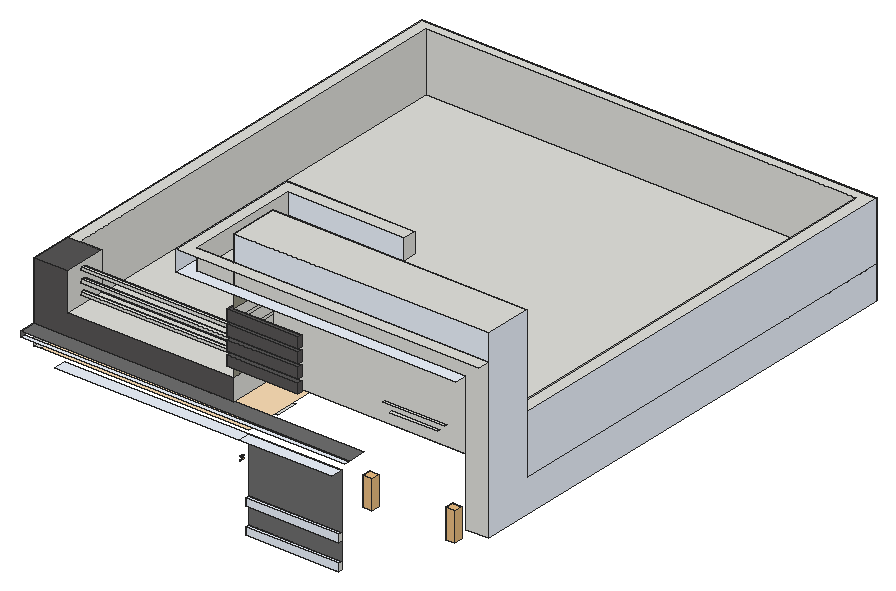
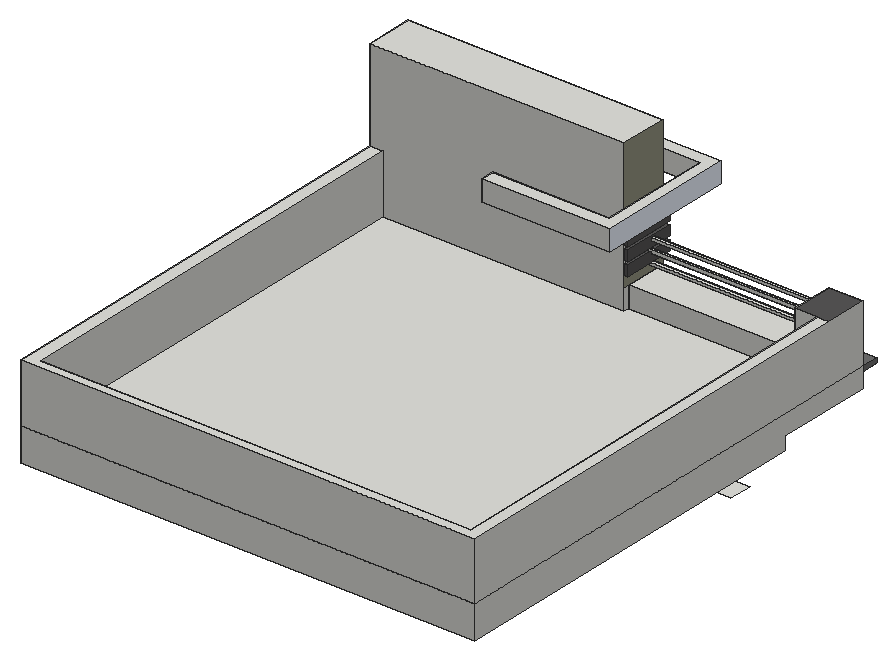
# SketchUp Ruby script. Lengths in inches.
U = 1.inch
M = Sketchup.active_model
def pt(a) = Geom::Point3d.new(a.map { |v| v * U })
def face(e, loops, mat)
  f = e.add_face(loops[0].map { |a| pt(a) })
  loops[1..].each { |l| e.add_face(l.map { |a| pt(a) }).erase! }
  f.material = f.back_material = mat if mat
  f
end
# faces: each face lists its corners as indices into pts; further lists are holes
def faces(e, pts, list, mat = nil) = list.each { |f| face(e, (f[0].is_a?(Array) ? f : [f]).map { |l| l.map { |i| pts[i] } }, mat) }
# xy, xz, yz: faces in a plane at the given z, y or x. An outline is a flat list of corners, or four numbers for a rectangle; further outlines are holes
def ring(l) = l.size == 4 ? [[l[0], l[1]], [l[2], l[1]], [l[2], l[3]], [l[0], l[3]]] : l.each_slice(2).to_a
def flat(e, list, mat, &to3) = list.each { |f| face(e, (f[0].is_a?(Array) ? f : [f]).map { |l| ring(l).map { |u, v| to3.(u, v) } }, mat) }
def xy(e, z, list, mat = nil) = flat(e, list, mat) { |x, y| [x, y, z] }
def xz(e, y, list, mat = nil) = flat(e, list, mat) { |x, z| [x, y, z] }
def yz(e, x, list, mat = nil) = flat(e, list, mat) { |y, z| [x, y, z] }
def lines(e, pts, list) = list.each { |a, b| e.add_line(pt(pts[a]), pt(pts[b])) }
# prism: a flat outline (further loops are holes) pulled along v
def prism(e, loops, v, mat = nil)
  f = face(e, loops, mat); d = Geom::Vector3d.new(v.map { |x| x * U })
  f.pushpull(f.normal.samedirection?(d) ? d.length : -d.length)
end
def box(e, o, s, mat = nil) = prism(e, [[o, [o[0] + s[0], o[1], o[2]], [o[0] + s[0], o[1] + s[1], o[2]], [o[0], o[1] + s[1], o[2]]]], [0, 0, s[2]], mat)
def at(x, y, z, deg = 0) = Geom::Transformation.translation(pt([x, y, z])) * Geom::Transformation.rotation(ORIGIN, Z_AXIS, deg.degrees)
def axes(o, x, y, z) = Geom::Transformation.new([*x, 0, *y, 0, *z, 0, *pt(o).to_a, 1])
def part(name) = M.definitions.add(name)
# library, detail: a bought-in or finely detailed component or shape, given as its bounding box
def library(name, o, s) = part(name).tap { |d| box(d.entities, o, s) }
def detail(e, o, s) = box(e.add_group.entities, o, s)
def put(e, d, t, mat = nil) = e.add_instance(d, t).tap { |i| i.material = mat if mat }
def group(e, t, mat = nil) = e.add_group.tap { |g| g.transformation = t; g.material = mat if mat }.entities
root = M.entities
M.materials.add("Generic").color = [111, 111, 111]
M.materials.add("Generic\#1").color = [88, 86, 86]
M.materials.add("Generic\#2").color = [253, 222, 182]
M.materials.add("Generic\#3").color = [151, 150, 132]
M.materials.add("Generic\#4").color = [238, 245, 255]
M.materials.add("Generic\#5").color = [7, 6, 6]
M.materials.add("Material \#1").color = [140, 140, 140]
c1 = library("3DGeom~14_Defintion",[-102.17,352.37,-727.27],[204.35,204.35,1000])
c2 = library("3DGeom~1_Defintion",[-60.87,347.29,-704.08],[121.74,121.75,1000])
c3 = library("Lamp Wall Outdoor 94-02",[-1.89,-4.65,-3.17],[3.78,4.65,6.35])
xy(root,197.069,[[128.435,116.314,128.381,116.332,128.4375,116.329],[128.435,116.314,128.4375,116.329,128.489,116.329],[128.435,116.314,128.489,116.329,128.492,116.314],[128.492,116.314,128.489,116.329,128.537,116.346],[128.492,116.314,128.537,116.346,128.545,116.332],
  [128.4375,116.329,128.381,116.332,128.389,116.346],[128.381,116.332,128.337,116.367,128.389,116.346],[128.545,116.332,128.537,116.346,128.576,116.377],[128.545,116.332,128.576,116.377,128.589,116.367],[128.389,116.346,128.337,116.367,128.35,116.377],
  [128.337,116.367,128.309,116.413,128.35,116.377],[128.589,116.367,128.576,116.377,128.602,116.418],[128.589,116.367,128.602,116.418,128.617,116.413],[128.35,116.377,128.309,116.413,128.324,116.418],[128.309,116.413,128.299,116.465,128.324,116.418],
  [128.617,116.413,128.602,116.418,128.611,116.465],[128.617,116.413,128.611,116.465,128.627,116.465],[128.324,116.418,128.299,116.465,128.315,116.465],[128.299,116.465,128.309,116.518,128.315,116.465],[128.315,116.465,128.309,116.518,128.324,116.513],
  [128.611,116.465,128.602,116.513,128.627,116.465],[128.627,116.465,128.602,116.513,128.617,116.518],[128.324,116.513,128.309,116.518,128.337,116.564],[128.324,116.513,128.337,116.564,128.35,116.554],[128.602,116.513,128.576,116.554,128.617,116.518],
  [128.617,116.518,128.576,116.554,128.589,116.564],[128.35,116.554,128.337,116.564,128.381,116.598],[128.35,116.554,128.381,116.598,128.389,116.585],[128.576,116.554,128.537,116.585,128.589,116.564],[128.589,116.564,128.537,116.585,128.545,116.598],
  [128.389,116.585,128.381,116.598,128.435,116.616],[128.389,116.585,128.435,116.616,128.4375,116.601],[128.537,116.585,128.489,116.601,128.545,116.598],[128.545,116.598,128.489,116.601,128.492,116.616],[128.4375,116.601,128.435,116.616,128.492,116.616],
  [128.4375,116.601,128.492,116.616,128.489,116.601]],"Material \#1")
xy(root,197.085,[[128.435,116.314,128.389,116.346,128.381,116.332],[128.435,116.314,128.4375,116.329,128.389,116.346],[128.435,116.314,128.492,116.314,128.4375,116.329],[128.492,116.314,128.489,116.329,128.4375,116.329],[128.492,116.314,128.545,116.332,128.489,116.329],
  [128.489,116.329,128.545,116.332,128.537,116.346],[128.381,116.332,128.35,116.377,128.337,116.367],[128.381,116.332,128.389,116.346,128.35,116.377],[128.545,116.332,128.589,116.367,128.537,116.346],[128.537,116.346,128.589,116.367,128.576,116.377],
  [128.337,116.367,128.324,116.418,128.309,116.413],[128.337,116.367,128.35,116.377,128.324,116.418],[128.589,116.367,128.617,116.413,128.576,116.377],[128.576,116.377,128.617,116.413,128.602,116.418],[128.309,116.413,128.315,116.465,128.299,116.465],
  [128.309,116.413,128.324,116.418,128.315,116.465],[128.617,116.413,128.627,116.465,128.602,116.418],[128.602,116.418,128.627,116.465,128.611,116.465],[128.299,116.465,128.315,116.465,128.324,116.513],[128.299,116.465,128.324,116.513,128.309,116.518],
  [128.611,116.465,128.617,116.518,128.602,116.513],[128.611,116.465,128.627,116.465,128.617,116.518],[128.324,116.513,128.35,116.554,128.309,116.518],[128.602,116.513,128.589,116.564,128.576,116.554],[128.602,116.513,128.617,116.518,128.589,116.564],
  [128.309,116.518,128.35,116.554,128.337,116.564],[128.35,116.554,128.389,116.585,128.337,116.564],[128.576,116.554,128.545,116.598,128.537,116.585],[128.576,116.554,128.589,116.564,128.545,116.598],[128.337,116.564,128.389,116.585,128.381,116.598],
  [128.389,116.585,128.4375,116.601,128.381,116.598],[128.537,116.585,128.492,116.616,128.489,116.601],[128.537,116.585,128.545,116.598,128.492,116.616],[128.381,116.598,128.4375,116.601,128.435,116.616],[128.4375,116.601,128.489,116.601,128.435,116.616],
  [128.489,116.601,128.492,116.616,128.435,116.616]],"Material \#1")
xy(root,203.189,[[169.979,34.653,243.692,37.591]],"Generic\#4")
xy(root,209.126,[[169.979,34.653,243.692,37.591]],"Generic\#4")
xy(root,223.751,[[169.979,34.653,243.692,37.591]],"Generic\#4")
xy(root,228.434,[[128.435,116.314,128.381,116.332,128.389,116.346],[128.435,116.314,128.389,116.346,128.4375,116.329],[128.435,116.314,128.4375,116.329,128.492,116.314],[128.492,116.314,128.4375,116.329,128.489,116.329],[128.492,116.314,128.489,116.329,128.545,116.332],
  [128.489,116.329,128.537,116.346,128.545,116.332],[128.381,116.332,128.337,116.367,128.35,116.377],[128.381,116.332,128.35,116.377,128.389,116.346],[128.545,116.332,128.537,116.346,128.589,116.367],[128.537,116.346,128.576,116.377,128.589,116.367],
  [128.337,116.367,128.309,116.413,128.324,116.418],[128.337,116.367,128.324,116.418,128.35,116.377],[128.589,116.367,128.576,116.377,128.617,116.413],[128.576,116.377,128.602,116.418,128.617,116.413],[128.309,116.413,128.299,116.465,128.315,116.465],
  [128.309,116.413,128.315,116.465,128.324,116.418],[128.617,116.413,128.602,116.418,128.627,116.465],[128.602,116.418,128.611,116.465,128.627,116.465],[128.299,116.465,128.309,116.518,128.324,116.513],[128.299,116.465,128.324,116.513,128.315,116.465],
  [128.611,116.465,128.602,116.513,128.617,116.518],[128.611,116.465,128.617,116.518,128.627,116.465],[128.324,116.513,128.309,116.518,128.35,116.554],[128.602,116.513,128.576,116.554,128.589,116.564],[128.602,116.513,128.589,116.564,128.617,116.518],
  [128.309,116.518,128.337,116.564,128.35,116.554],[128.35,116.554,128.337,116.564,128.389,116.585],[128.576,116.554,128.537,116.585,128.545,116.598],[128.576,116.554,128.545,116.598,128.589,116.564],[128.337,116.564,128.381,116.598,128.389,116.585],
  [128.389,116.585,128.381,116.598,128.4375,116.601],[128.537,116.585,128.489,116.601,128.492,116.616],[128.537,116.585,128.492,116.616,128.545,116.598],[128.381,116.598,128.435,116.616,128.4375,116.601],[128.4375,116.601,128.435,116.616,128.489,116.601],
  [128.489,116.601,128.435,116.616,128.492,116.616]],"Material \#1")
xy(root,228.449,[[128.435,116.314,128.4375,116.329,128.381,116.332],[128.435,116.314,128.489,116.329,128.4375,116.329],[128.435,116.314,128.492,116.314,128.489,116.329],[128.492,116.314,128.537,116.346,128.489,116.329],[128.492,116.314,128.545,116.332,128.537,116.346],
  [128.4375,116.329,128.389,116.346,128.381,116.332],[128.381,116.332,128.389,116.346,128.337,116.367],[128.545,116.332,128.576,116.377,128.537,116.346],[128.545,116.332,128.589,116.367,128.576,116.377],[128.389,116.346,128.35,116.377,128.337,116.367],
  [128.337,116.367,128.35,116.377,128.309,116.413],[128.589,116.367,128.602,116.418,128.576,116.377],[128.589,116.367,128.617,116.413,128.602,116.418],[128.35,116.377,128.324,116.418,128.309,116.413],[128.309,116.413,128.324,116.418,128.299,116.465],
  [128.617,116.413,128.611,116.465,128.602,116.418],[128.617,116.413,128.627,116.465,128.611,116.465],[128.324,116.418,128.315,116.465,128.299,116.465],[128.299,116.465,128.315,116.465,128.309,116.518],[128.315,116.465,128.324,116.513,128.309,116.518],
  [128.611,116.465,128.627,116.465,128.602,116.513],[128.627,116.465,128.617,116.518,128.602,116.513],[128.324,116.513,128.337,116.564,128.309,116.518],[128.324,116.513,128.35,116.554,128.337,116.564],[128.602,116.513,128.617,116.518,128.576,116.554],
  [128.617,116.518,128.589,116.564,128.576,116.554],[128.35,116.554,128.381,116.598,128.337,116.564],[128.35,116.554,128.389,116.585,128.381,116.598],[128.576,116.554,128.589,116.564,128.537,116.585],[128.589,116.564,128.545,116.598,128.537,116.585],
  [128.389,116.585,128.435,116.616,128.381,116.598],[128.389,116.585,128.4375,116.601,128.435,116.616],[128.537,116.585,128.545,116.598,128.489,116.601],[128.545,116.598,128.492,116.616,128.489,116.601],[128.4375,116.601,128.492,116.616,128.435,116.616],
  [128.4375,116.601,128.489,116.601,128.492,116.616]],"Material \#1")
xy(root,229.689,[[169.979,34.653,243.692,37.591]],"Generic\#4")
xy(root,231.472,[[27.868,114.716,69.368,133.091]])
xy(root,231.923,[[128.435,116.314,128.381,116.332,128.4375,116.329],[128.435,116.314,128.4375,116.329,128.489,116.329],[128.435,116.314,128.489,116.329,128.492,116.314],[128.492,116.314,128.489,116.329,128.537,116.346],[128.492,116.314,128.537,116.346,128.545,116.332],
  [128.4375,116.329,128.381,116.332,128.389,116.346],[128.381,116.332,128.337,116.367,128.389,116.346],[128.545,116.332,128.537,116.346,128.576,116.377],[128.545,116.332,128.576,116.377,128.589,116.367],[128.389,116.346,128.337,116.367,128.35,116.377],
  [128.337,116.367,128.309,116.413,128.35,116.377],[128.589,116.367,128.576,116.377,128.602,116.418],[128.589,116.367,128.602,116.418,128.617,116.413],[128.35,116.377,128.309,116.413,128.324,116.418],[128.309,116.413,128.299,116.465,128.324,116.418],
  [128.617,116.413,128.602,116.418,128.611,116.465],[128.617,116.413,128.611,116.465,128.627,116.465],[128.324,116.418,128.299,116.465,128.315,116.465],[128.299,116.465,128.309,116.518,128.315,116.465],[128.315,116.465,128.309,116.518,128.324,116.513],
  [128.611,116.465,128.602,116.513,128.627,116.465],[128.627,116.465,128.602,116.513,128.617,116.518],[128.324,116.513,128.309,116.518,128.337,116.564],[128.324,116.513,128.337,116.564,128.35,116.554],[128.602,116.513,128.576,116.554,128.617,116.518],
  [128.617,116.518,128.576,116.554,128.589,116.564],[128.35,116.554,128.337,116.564,128.381,116.598],[128.35,116.554,128.381,116.598,128.389,116.585],[128.576,116.554,128.537,116.585,128.589,116.564],[128.589,116.564,128.537,116.585,128.545,116.598],
  [128.389,116.585,128.381,116.598,128.435,116.616],[128.389,116.585,128.435,116.616,128.4375,116.601],[128.537,116.585,128.489,116.601,128.545,116.598],[128.545,116.598,128.489,116.601,128.492,116.616],[128.4375,116.601,128.435,116.616,128.492,116.616],
  [128.4375,116.601,128.492,116.616,128.489,116.601]],"Material \#1")
xy(root,231.939,[[128.435,116.314,128.389,116.346,128.381,116.332],[128.435,116.314,128.4375,116.329,128.389,116.346],[128.435,116.314,128.492,116.314,128.4375,116.329],[128.492,116.314,128.489,116.329,128.4375,116.329],[128.492,116.314,128.545,116.332,128.489,116.329],
  [128.489,116.329,128.545,116.332,128.537,116.346],[128.381,116.332,128.35,116.377,128.337,116.367],[128.381,116.332,128.389,116.346,128.35,116.377],[128.545,116.332,128.589,116.367,128.537,116.346],[128.537,116.346,128.589,116.367,128.576,116.377],
  [128.337,116.367,128.324,116.418,128.309,116.413],[128.337,116.367,128.35,116.377,128.324,116.418],[128.589,116.367,128.617,116.413,128.576,116.377],[128.576,116.377,128.617,116.413,128.602,116.418],[128.309,116.413,128.315,116.465,128.299,116.465],
  [128.309,116.413,128.324,116.418,128.315,116.465],[128.617,116.413,128.627,116.465,128.602,116.418],[128.602,116.418,128.627,116.465,128.611,116.465],[128.299,116.465,128.315,116.465,128.324,116.513],[128.299,116.465,128.324,116.513,128.309,116.518],
  [128.611,116.465,128.617,116.518,128.602,116.513],[128.611,116.465,128.627,116.465,128.617,116.518],[128.324,116.513,128.35,116.554,128.309,116.518],[128.602,116.513,128.589,116.564,128.576,116.554],[128.602,116.513,128.617,116.518,128.589,116.564],
  [128.309,116.518,128.35,116.554,128.337,116.564],[128.35,116.554,128.389,116.585,128.337,116.564],[128.576,116.554,128.545,116.598,128.537,116.585],[128.576,116.554,128.589,116.564,128.545,116.598],[128.337,116.564,128.389,116.585,128.381,116.598],
  [128.389,116.585,128.4375,116.601,128.381,116.598],[128.537,116.585,128.492,116.616,128.489,116.601],[128.537,116.585,128.545,116.598,128.492,116.616],[128.381,116.598,128.4375,116.601,128.435,116.616],[128.4375,116.601,128.489,116.601,128.435,116.616],
  [128.489,116.601,128.492,116.616,128.435,116.616]],"Material \#1")
xy(root,239.461,[[95.815,114.716,131.252,133.091]])
xy(root,273.875,[[24.805,27.716,169.979,37.591],[169.979,27.716,243.692,37.591]],"Generic\#4")
xy(root,276.8125,[[0,37.591,5.4375,114.716]])
xy(root,276.8125,[[5.4375,37.591,169.979,114.716]],"Generic\#2")
xy(root,288.8125,[[0,24.153,257.286,27.716]],"Generic\#4")
xy(root,292.75,[[0,37.591,0,421.591,360,421.591,360,75.716,349.8125,75.716,349.8125,414.278,9.125,414.278,9.125,71.216,158.474,71.216,158.474,37.591],[9.125,71.216,158.474,71.216,158.474,75.716,349.8125,75.716,349.8125,414.278,9.125,414.278]])
xy(root,292.75,[[0,24.153,260.974,37.591]],"Generic")
xy(root,309.4375,[[26.756,37.591,158.474,71.216]])
xy(root,318.275,[[155.536,34.341,155.536,75.716,158.474,75.716,158.474,37.591,211.974,37.591,211.974,34.341]],"Generic\#1")
xy(root,326.4,[[155.536,34.341,211.974,34.341,211.974,37.591,158.474,37.591,158.474,75.716,155.536,75.716]],"Generic\#1")
xy(root,329.025,[[155.536,34.341,155.536,75.716,158.474,75.716,158.474,37.591,211.974,37.591,211.974,34.341]],"Generic\#1")
xy(root,329.742,[[283.712,35.716,321.15,37.591]])
xy(root,335.362,[[278.093,35.716,326.77,37.591]])
xy(root,337.15,[[155.536,34.341,211.974,34.341,211.974,37.591,158.474,37.591,158.474,75.716,155.536,75.716]],"Generic\#1")
xy(root,339.0625,[[0,71.216,9.125,71.216,9.125,414.278,349.8125,414.278,349.8125,75.716,360,75.716,360,421.591,0,421.591]])
xy(root,339.0625,[[0,37.591,26.756,71.216]],"Generic\#1")
xy(root,339.775,[[155.536,34.341,155.536,75.716,158.474,75.716,158.474,37.591,211.974,37.591,211.974,34.341]],"Generic\#1")
xy(root,347.9,[[155.536,34.341,211.974,34.341,211.974,37.591,158.474,37.591,158.474,75.716,155.536,75.716]],"Generic\#1")
xy(root,350.4,[[155.536,34.341,155.536,75.716,158.474,75.716,158.474,37.591,211.974,37.591,211.974,34.341]],"Generic\#1")
xy(root,358.525,[[155.536,34.341,211.974,34.341,211.974,37.591,158.474,37.591,158.474,75.716,155.536,75.716]],"Generic\#1")
xy(root,375.448,[[120.099,27.716,120.099,137.653,221.7,137.653,221.7,126.966,129.325,126.966,129.325,37.591,342.12,37.591,342.12,27.716]],"Generic\#4")
xy(root,391.636,[[120.099,27.716,360,27.716,360,37.591,129.325,37.591,129.325,126.966,221.7,126.966,221.7,137.653,120.099,137.653]])
xy(root,411.9375,[[158.474,37.591,360,75.716]])
xz(root,34.341,[[155.536,318.275,211.974,326.4],[155.536,329.025,211.974,337.15],[155.536,339.775,211.974,347.9],[155.536,350.4,211.974,358.525]],"Generic\#1")
xz(root,34.653,[[169.979,203.189,243.692,209.126],[169.979,223.751,243.692,229.689]],"Generic\#4")
xz(root,37.591,[[169.979,203.189,243.692,209.126],[169.979,223.751,243.692,229.689],[342.12,266.375,342.12,375.448,158.474,375.448,158.474,391.636,360,391.636,360,266.375],[158.474,318.275,211.974,326.4],[158.474,329.025,211.974,337.15],
  [158.474,339.775,211.974,347.9],[158.474,350.4,211.974,358.525],[129.325,375.448,158.474,391.636]])
xz(root,37.591,[[169.979,209.126,243.692,223.751],[169.979,229.689,243.692,273.875]],"Generic")
xz(root,37.591,[[0,292.75,158.474,292.75,158.474,309.4375,26.756,309.4375,26.756,339.0625,0,339.0625]],"Generic\#1")
xz(root,37.591,[[158.474,391.636,360,411.9375]],"Generic\#4")
xz(root,50.453,[[26.756,333.876,158.474,336.189]])
xz(root,50.515,[[26.756,316.376,158.474,318.689]])
xz(root,50.578,[[26.756,325.126,158.474,327.439]])
xz(root,53.135,[[26.756,334.072,158.474,336.384]])
xz(root,53.197,[[26.756,316.572,158.474,318.884]])
xz(root,53.26,[[26.756,325.322,158.474,327.634]])
xz(root,71.216,[[9.125,292.75,9.125,339.0625,26.756,339.0625,26.756,309.4375,158.474,309.4375,158.474,292.75]])
xz(root,75.716,[[158.474,292.75,158.474,411.9375,360,411.9375,360,339.0625,349.8125,339.0625,349.8125,292.75]])
xz(root,75.716,[[155.536,318.275,158.474,326.4],[155.536,329.025,158.474,337.15],[155.536,339.775,158.474,347.9],[155.536,350.4,158.474,358.525]],"Generic\#1")
xz(root,115.852,[[100.819,199.181,100.828,199.308,100.828,199.181],[100.828,199.181,100.828,199.308,100.838,199.305],[101.957,199.181,101.948,199.305,101.967,199.181],[101.967,199.181,101.948,199.305,101.957,199.308],[101.393,199.232,101.359,199.235,101.393,199.243],
  [101.393,199.232,101.393,199.243,101.425,199.247],[101.393,199.232,101.425,199.247,101.427,199.235],[101.359,199.235,101.326,199.246,101.36,199.247],[101.359,199.235,101.36,199.247,101.393,199.243],[101.427,199.235,101.425,199.247,101.456,199.257],
  [101.427,199.235,101.456,199.257,101.459,199.246],[101.326,199.246,101.297,199.263,101.33,199.257],[101.326,199.246,101.33,199.257,101.36,199.247],[101.459,199.246,101.456,199.257,101.484,199.273],[101.459,199.246,101.484,199.273,101.489,199.263],
  [101.33,199.257,101.297,199.263,101.302,199.273],[101.297,199.263,101.27,199.285,101.302,199.273],[101.489,199.263,101.484,199.273,101.509,199.294],[101.489,199.263,101.509,199.294,101.516,199.285],[101.302,199.273,101.27,199.285,101.276,199.294],
  [101.27,199.285,101.247,199.312,101.276,199.294],[101.516,199.285,101.509,199.294,101.531,199.319],[101.516,199.285,101.531,199.319,101.539,199.312],[101.276,199.294,101.247,199.312,101.255,199.319],[100.838,199.305,100.828,199.308,100.855,199.422],
  [100.838,199.305,100.855,199.422,100.864,199.418],[101.948,199.305,101.921,199.418,101.957,199.308],[101.957,199.308,101.921,199.418,101.931,199.422],[101.247,199.312,101.228,199.343,101.255,199.319],[101.539,199.312,101.531,199.319,101.549,199.349],
  [101.539,199.312,101.549,199.349,101.557,199.343],[101.255,199.319,101.228,199.343,101.237,199.349],[101.228,199.343,101.214,199.378,101.237,199.349],[101.557,199.343,101.549,199.349,101.562,199.382],[101.557,199.343,101.562,199.382,101.571,199.378],
  [101.237,199.349,101.214,199.378,101.223,199.382],[101.214,199.378,101.205,199.417,101.223,199.382],[101.571,199.378,101.562,199.382,101.571,199.419],[101.571,199.378,101.571,199.419,101.58,199.417],[101.223,199.382,101.205,199.417,101.215,199.419],
  [101.205,199.417,101.202,199.467,101.215,199.419],[101.58,199.417,101.571,199.419,101.574,199.457],[101.58,199.417,101.574,199.457,101.583,199.457],[100.864,199.418,100.855,199.422,100.897,199.527],[100.864,199.418,100.897,199.527,100.906,199.521],
  [101.921,199.418,101.88,199.521,101.931,199.422],[101.215,199.419,101.202,199.467,101.212,199.467],[101.931,199.422,101.88,199.521,101.888,199.527],[101.574,199.457,101.571,199.495,101.583,199.457],[101.583,199.457,101.571,199.495,101.58,199.497],
  [101.202,199.467,101.205,199.497,101.212,199.467],[101.212,199.467,101.205,199.497,101.215,199.495],[101.215,199.495,101.205,199.497,101.214,199.535],[101.215,199.495,101.214,199.535,101.223,199.531],[101.571,199.495,101.562,199.531,101.58,199.497],
  [101.58,199.497,101.562,199.531,101.571,199.535],[100.906,199.521,100.897,199.527,100.956,199.625],[100.906,199.521,100.956,199.625,100.964,199.618],[101.88,199.521,101.824,199.614,101.888,199.527],[101.888,199.527,101.824,199.614,101.832,199.622],
  [101.223,199.531,101.214,199.535,101.228,199.57],[101.223,199.531,101.228,199.57,101.237,199.565],[101.562,199.531,101.549,199.565,101.571,199.535],[101.571,199.535,101.549,199.565,101.557,199.57],[101.237,199.565,101.228,199.57,101.247,199.602],
  [101.237,199.565,101.247,199.602,101.255,199.594],[101.549,199.565,101.531,199.594,101.557,199.57],[101.557,199.57,101.531,199.594,101.539,199.602],[101.255,199.594,101.247,199.602,101.27,199.629],[101.255,199.594,101.27,199.629,101.276,199.62],
  [101.531,199.594,101.509,199.62,101.539,199.602],[101.539,199.602,101.509,199.62,101.516,199.629],[101.824,199.614,101.756,199.695,101.832,199.622],[100.964,199.618,100.956,199.625,101.023,199.704],[100.964,199.618,101.023,199.704,101.03,199.695],
  [101.276,199.62,101.27,199.629,101.297,199.651],[101.276,199.62,101.297,199.651,101.302,199.641],[101.509,199.62,101.484,199.641,101.516,199.629],[101.832,199.622,101.756,199.695,101.762,199.704],[101.516,199.629,101.484,199.641,101.489,199.651],
  [101.302,199.641,101.297,199.651,101.326,199.668],[101.302,199.641,101.326,199.668,101.33,199.657],[101.484,199.641,101.456,199.657,101.489,199.651],[101.489,199.651,101.456,199.657,101.459,199.668],[101.33,199.657,101.326,199.668,101.359,199.678],
  [101.33,199.657,101.359,199.678,101.36,199.667],[101.456,199.657,101.425,199.667,101.459,199.668],[101.36,199.667,101.359,199.678,101.393,199.682],[101.36,199.667,101.393,199.682,101.393,199.67],[101.425,199.667,101.393,199.67,101.427,199.678],
  [101.425,199.667,101.427,199.678,101.459,199.668],[101.393,199.67,101.393,199.682,101.427,199.678],[101.03,199.695,101.023,199.704,101.103,199.771],[101.03,199.695,101.103,199.771,101.108,199.76],[101.756,199.695,101.677,199.76,101.762,199.704],
  [101.762,199.704,101.677,199.76,101.682,199.771],[101.108,199.76,101.103,199.771,101.193,199.821],[101.108,199.76,101.193,199.821,101.196,199.81],[101.677,199.76,101.589,199.81,101.682,199.771],[101.682,199.771,101.589,199.81,101.593,199.821],
  [101.196,199.81,101.193,199.821,101.29,199.852],[101.196,199.81,101.29,199.852,101.291,199.841],[101.589,199.81,101.494,199.841,101.593,199.821],[101.593,199.821,101.494,199.841,101.496,199.852],[101.291,199.841,101.29,199.852,101.393,199.863],
  [101.291,199.841,101.393,199.863,101.393,199.851],[101.494,199.841,101.393,199.851,101.496,199.852],[101.393,199.851,101.393,199.863,101.496,199.852]],"Material \#1")
xz(root,117.632,[[100.819,199.181,100.828,199.181,100.828,199.308],[100.828,199.181,100.838,199.305,100.828,199.308],[101.957,199.181,101.967,199.181,101.948,199.305],[101.967,199.181,101.957,199.308,101.948,199.305],[101.393,199.232,101.393,199.243,101.359,199.235],
  [101.393,199.232,101.425,199.247,101.393,199.243],[101.393,199.232,101.427,199.235,101.425,199.247],[101.359,199.235,101.36,199.247,101.326,199.246],[101.359,199.235,101.393,199.243,101.36,199.247],[101.427,199.235,101.456,199.257,101.425,199.247],
  [101.427,199.235,101.459,199.246,101.456,199.257],[101.326,199.246,101.33,199.257,101.297,199.263],[101.326,199.246,101.36,199.247,101.33,199.257],[101.459,199.246,101.484,199.273,101.456,199.257],[101.459,199.246,101.489,199.263,101.484,199.273],
  [101.33,199.257,101.302,199.273,101.297,199.263],[101.297,199.263,101.302,199.273,101.27,199.285],[101.489,199.263,101.509,199.294,101.484,199.273],[101.489,199.263,101.516,199.285,101.509,199.294],[101.302,199.273,101.276,199.294,101.27,199.285],
  [101.27,199.285,101.276,199.294,101.247,199.312],[101.516,199.285,101.531,199.319,101.509,199.294],[101.516,199.285,101.539,199.312,101.531,199.319],[101.276,199.294,101.255,199.319,101.247,199.312],[100.838,199.305,100.855,199.422,100.828,199.308],
  [100.838,199.305,100.864,199.418,100.855,199.422],[101.948,199.305,101.957,199.308,101.921,199.418],[101.957,199.308,101.931,199.422,101.921,199.418],[101.247,199.312,101.255,199.319,101.228,199.343],[101.539,199.312,101.549,199.349,101.531,199.319],
  [101.539,199.312,101.557,199.343,101.549,199.349],[101.255,199.319,101.237,199.349,101.228,199.343],[101.228,199.343,101.237,199.349,101.214,199.378],[101.557,199.343,101.562,199.382,101.549,199.349],[101.557,199.343,101.571,199.378,101.562,199.382],
  [101.237,199.349,101.223,199.382,101.214,199.378],[101.214,199.378,101.223,199.382,101.205,199.417],[101.571,199.378,101.571,199.419,101.562,199.382],[101.571,199.378,101.58,199.417,101.571,199.419],[101.223,199.382,101.215,199.419,101.205,199.417],
  [101.205,199.417,101.215,199.419,101.202,199.467],[101.58,199.417,101.574,199.457,101.571,199.419],[101.58,199.417,101.583,199.457,101.574,199.457],[100.864,199.418,100.897,199.527,100.855,199.422],[100.864,199.418,100.906,199.521,100.897,199.527],
  [101.921,199.418,101.931,199.422,101.88,199.521],[101.215,199.419,101.212,199.467,101.202,199.467],[101.931,199.422,101.888,199.527,101.88,199.521],[101.574,199.457,101.583,199.457,101.571,199.495],[101.583,199.457,101.58,199.497,101.571,199.495],
  [101.202,199.467,101.212,199.467,101.205,199.497],[101.212,199.467,101.215,199.495,101.205,199.497],[101.215,199.495,101.214,199.535,101.205,199.497],[101.215,199.495,101.223,199.531,101.214,199.535],[101.571,199.495,101.58,199.497,101.562,199.531],
  [101.58,199.497,101.571,199.535,101.562,199.531],[100.906,199.521,100.956,199.625,100.897,199.527],[100.906,199.521,100.964,199.618,100.956,199.625],[101.88,199.521,101.888,199.527,101.824,199.614],[101.888,199.527,101.832,199.622,101.824,199.614],
  [101.223,199.531,101.228,199.57,101.214,199.535],[101.223,199.531,101.237,199.565,101.228,199.57],[101.562,199.531,101.571,199.535,101.549,199.565],[101.571,199.535,101.557,199.57,101.549,199.565],[101.237,199.565,101.247,199.602,101.228,199.57],
  [101.237,199.565,101.255,199.594,101.247,199.602],[101.549,199.565,101.557,199.57,101.531,199.594],[101.557,199.57,101.539,199.602,101.531,199.594],[101.255,199.594,101.27,199.629,101.247,199.602],[101.255,199.594,101.276,199.62,101.27,199.629],
  [101.531,199.594,101.539,199.602,101.509,199.62],[101.539,199.602,101.516,199.629,101.509,199.62],[101.824,199.614,101.832,199.622,101.756,199.695],[100.964,199.618,101.023,199.704,100.956,199.625],[100.964,199.618,101.03,199.695,101.023,199.704],
  [101.276,199.62,101.297,199.651,101.27,199.629],[101.276,199.62,101.302,199.641,101.297,199.651],[101.509,199.62,101.516,199.629,101.484,199.641],[101.832,199.622,101.762,199.704,101.756,199.695],[101.516,199.629,101.489,199.651,101.484,199.641],
  [101.302,199.641,101.326,199.668,101.297,199.651],[101.302,199.641,101.33,199.657,101.326,199.668],[101.484,199.641,101.489,199.651,101.456,199.657],[101.489,199.651,101.459,199.668,101.456,199.657],[101.33,199.657,101.359,199.678,101.326,199.668],
  [101.33,199.657,101.36,199.667,101.359,199.678],[101.456,199.657,101.459,199.668,101.425,199.667],[101.36,199.667,101.393,199.682,101.359,199.678],[101.36,199.667,101.393,199.67,101.393,199.682],[101.425,199.667,101.427,199.678,101.393,199.67],
  [101.425,199.667,101.459,199.668,101.427,199.678],[101.393,199.67,101.427,199.678,101.393,199.682],[101.03,199.695,101.103,199.771,101.023,199.704],[101.03,199.695,101.108,199.76,101.103,199.771],[101.756,199.695,101.762,199.704,101.677,199.76],
  [101.762,199.704,101.682,199.771,101.677,199.76],[101.108,199.76,101.193,199.821,101.103,199.771],[101.108,199.76,101.196,199.81,101.193,199.821],[101.677,199.76,101.682,199.771,101.589,199.81],[101.682,199.771,101.593,199.821,101.589,199.81],
  [101.196,199.81,101.29,199.852,101.193,199.821],[101.196,199.81,101.291,199.841,101.29,199.852],[101.589,199.81,101.593,199.821,101.494,199.841],[101.593,199.821,101.496,199.852,101.494,199.841],[101.291,199.841,101.393,199.863,101.29,199.852],
  [101.291,199.841,101.393,199.851,101.393,199.863],[101.494,199.841,101.496,199.852,101.393,199.851],[101.393,199.851,101.496,199.852,101.393,199.863]],"Material \#1")
xz(root,126.966,[[129.325,375.448,221.7,391.636]],"Generic\#4")
xz(root,137.653,[[120.099,375.448,221.7,391.636]])
xz(root,414.278,[[9.125,292.75,349.8125,339.0625]])
xz(root,421.591,[[0,266.375,360,292.75],[0,292.75,360,339.0625]])
yz(root,0,[[114.716,266.375,114.716,276.8125,37.591,276.8125,37.591,292.75,421.591,292.75,421.591,266.375],[37.591,292.75,421.591,339.0625]])
yz(root,0,[[24.153,288.8125,37.591,292.75]],"Generic")
yz(root,9.125,[[71.216,292.75,414.278,339.0625]])
yz(root,26.756,[[[37.591,309.4375,71.216,339.0625],[50.453,333.876,50.453,336.189,53.135,336.384,53.135,334.072],[50.578,325.126,50.578,327.439,53.26,327.634,53.26,325.322],[50.515,316.376,50.515,318.689,53.197,318.884,53.197,316.572]],[50.515,316.376,50.515,318.689,53.197,318.884,53.197,316.572],[50.578,325.126,50.578,327.439,53.26,327.634,53.26,325.322],[50.453,333.876,50.453,336.189,53.135,336.384,53.135,334.072]])
yz(root,120.099,[[27.716,375.448,137.653,391.636]],"Generic\#4")
yz(root,129.325,[[37.591,375.448,126.966,391.636]])
yz(root,155.536,[[34.341,318.275,75.716,326.4],[34.341,329.025,75.716,337.15],[34.341,339.775,75.716,347.9],[34.341,350.4,75.716,358.525]],"Generic\#1")
yz(root,158.474,[[37.591,292.75,71.216,309.4375],[71.216,292.75,75.716,309.4375],[37.591,318.275,37.591,326.4,50.578,326.4,50.578,325.126,53.26,325.322,53.26,326.4,75.716,326.4,75.716,318.275,53.197,318.275,53.197,318.884,50.515,318.689,50.515,318.275],[50.515,318.275,53.197,318.275,53.197,318.884,50.515,318.689],[50.578,325.126,53.26,325.322,53.26,326.4,50.578,326.4],
  [37.591,326.4,37.591,329.025,75.716,329.025,75.716,326.4,53.26,326.4,53.26,327.634,50.578,327.439,50.578,326.4],[[37.591,329.025,75.716,337.15],[50.453,333.876,53.135,334.072,53.135,336.384,50.453,336.189]],[37.591,337.15,75.716,339.775],[37.591,339.775,75.716,347.9],[37.591,347.9,75.716,350.4],
  [37.591,350.4,75.716,358.525]])
yz(root,158.474,[[37.591,309.4375,37.591,318.275,50.515,318.275,50.515,316.376,53.197,316.572,53.197,318.275,75.716,318.275,75.716,309.4375],[37.591,358.525,75.716,411.9375]],"Generic\#3")
yz(root,169.979,[[34.653,203.189,37.591,209.126],[34.653,223.751,37.591,229.689]],"Generic\#4")
yz(root,211.974,[[34.341,318.275,37.591,326.4],[34.341,329.025,37.591,337.15],[34.341,339.775,37.591,347.9],[34.341,350.4,37.591,358.525]],"Generic\#1")
yz(root,221.7,[[126.966,375.448,137.653,391.636]])
yz(root,243.692,[[34.653,203.189,37.591,209.126],[34.653,223.751,37.591,229.689]])
yz(root,349.8125,[[75.716,292.75,414.278,339.0625]])
yz(root,360,[[37.591,266.375,421.591,266.375,421.591,292.75,75.716,292.75,75.716,411.9375,37.591,411.9375],[75.716,292.75,421.591,339.0625]],"Generic\#4")
p = [[101.415,115.851,199.359],[101.415,115.876,199.359],[101.428,115.882,199.333],[101.428,115.858,199.333],[101.448,115.882,199.343],[101.448,115.858,199.343],
  [101.466,115.882,199.36],[101.466,115.858,199.36],[101.415,117.632,199.359],[101.428,117.625,199.333],[101.428,117.601,199.333],[101.415,117.607,199.359],
  [101.448,117.625,199.343],[101.448,117.601,199.343],[101.466,117.625,199.36],[101.466,117.601,199.36],[101.343,115.849,199.506],[101.343,115.873,199.506],
  [101.404,115.873,199.382],[101.404,115.849,199.382],[101.442,115.873,199.408],[101.442,115.849,199.408],[101.454,115.851,199.385],[101.382,115.873,199.532],
  [101.382,115.849,199.532],[101.454,115.876,199.385],[101.343,117.634,199.506],[101.404,117.634,199.382],[101.404,117.61,199.382],[101.343,117.61,199.506],
  [101.454,117.632,199.385],[101.442,117.634,199.408],[101.442,117.61,199.408],[101.454,117.607,199.385],[101.382,117.634,199.532],[101.382,117.61,199.532],
  [101.332,115.851,199.529],[101.371,115.876,199.555],[101.371,115.851,199.555],[101.319,115.858,199.554],[101.319,115.882,199.554],[101.332,115.876,199.529],
  [101.319,117.625,199.554],[101.332,117.632,199.529],[101.332,117.607,199.529],[101.319,117.601,199.554],[101.371,117.632,199.555],[101.371,117.607,199.555],
  [101.358,115.858,199.58],[101.358,115.882,199.58],[101.337,115.882,199.57],[101.337,115.858,199.57],[101.358,117.625,199.58],[101.337,117.625,199.57],
  [101.337,117.601,199.57],[101.358,117.601,199.58],[26.756,50.515,316.376],[26.756,53.197,316.572],[158.474,53.197,316.572],[158.474,50.515,316.376],
  [26.756,53.197,318.884],[26.756,50.515,318.689],[158.474,50.515,318.689],[158.474,53.197,318.884],[26.756,50.578,325.126],[26.756,53.26,325.322],
  [158.474,53.26,325.322],[158.474,50.578,325.126],[26.756,53.26,327.634],[26.756,50.578,327.439],[158.474,50.578,327.439],[158.474,53.26,327.634],
  [26.756,50.453,333.876],[26.756,53.135,334.072],[158.474,53.135,334.072],[158.474,50.453,333.876],[26.756,53.135,336.384],[26.756,50.453,336.189],
  [158.474,50.453,336.189],[158.474,53.135,336.384],[26.756,51.685,335.444],[158.474,51.685,335.444],[26.756,51.685,326.506],[158.474,51.685,326.506],
  [26.756,51.685,317.569],[158.474,51.685,317.569]]
faces(root,p,[[0,1,2],[2,3,0],[3,2,4],[4,5,3],[5,4,6],[6,7,5],[8,9,10],[10,11,8],
  [9,12,13],[13,10,9],[12,14,15],[15,13,12],[16,17,18],[18,19,16],[19,18,1],[1,0,19],
  [20,21,22],[21,20,23],[23,24,21],[22,25,20],[7,6,25],[25,22,7],[26,27,28],[28,29,26],
  [27,8,11],[11,28,27],[30,31,32],[32,33,30],[31,34,35],[35,32,31],[14,30,33],[33,15,14],
  [17,16,36],[24,23,37],[37,38,24],[39,40,41],[41,36,39],[36,41,17],[42,43,44],[44,45,42],
  [43,26,29],[29,44,43],[34,46,47],[47,35,34],[48,49,50],[50,51,48],[51,50,40],[40,39,51],
  [38,37,49],[49,48,38],[52,53,54],[54,55,52],[53,42,45],[45,54,53],[46,52,55],[55,47,46]],"Material \#1")
faces(root,p,[[56,57,58,59],[60,61,62,63],[64,65,66,67],[68,69,70,71],[72,73,74,75],[76,77,78,79]])
lines(root,p,[[80,81],[82,83],[84,85]])
put(root,c1,axes([101.39,117.36,195.3125],[0.00289,0,0],[0,0,0.00341],[0,0.0027,0]),"Material \#1")
put(root,c2,axes([101.39,117.36,195.3125],[0.00322,0,0],[0,0,0.0038],[0,0.00301,0]),"Material \#1")
put(root,c3,axes([335.13,37.59,269.875],[1.9536,0,0],[0,1.48,0],[0,0,3.6112]),"Generic\#5")
put(root,c3,axes([269.82,37.59,269.875],[1.9536,0,0],[0,1.48,0],[0,0,3.6112]),"Generic\#5")
